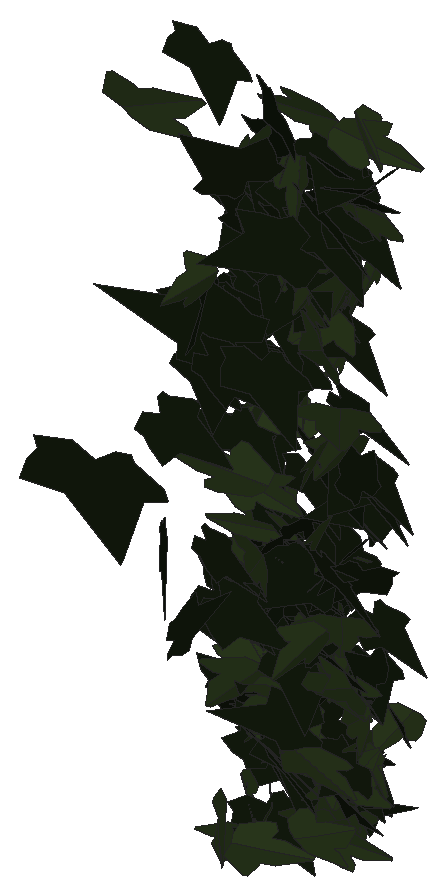
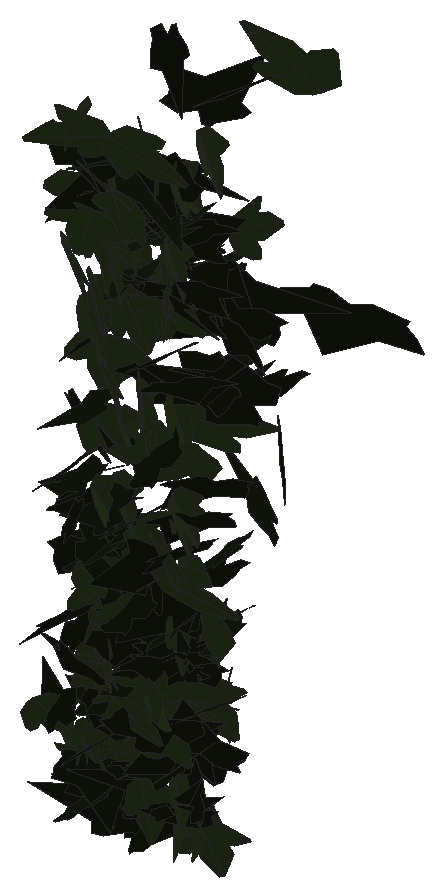
# SketchUp Ruby script. Lengths in millimetres.
U = 1.mm
M = Sketchup.active_model
def pt(a) = Geom::Point3d.new(a.map { |v| v * U })
def face(e, loops, mat)
  f = e.add_face(loops[0].map { |a| pt(a) })
  loops[1..].each { |l| e.add_face(l.map { |a| pt(a) }).erase! }
  f.material = f.back_material = mat if mat
  f
end
# faces: each face lists its corners as indices into pts; further lists are holes
def faces(e, pts, list, mat = nil) = list.each { |f| face(e, (f[0].is_a?(Array) ? f : [f]).map { |l| l.map { |i| pts[i] } }, mat) }
# xy, xz, yz: faces in a plane at the given z, y or x. An outline is a flat list of corners, or four numbers for a rectangle; further outlines are holes
def ring(l) = l.size == 4 ? [[l[0], l[1]], [l[2], l[1]], [l[2], l[3]], [l[0], l[3]]] : l.each_slice(2).to_a
def flat(e, list, mat, &to3) = list.each { |f| face(e, (f[0].is_a?(Array) ? f : [f]).map { |l| ring(l).map { |u, v| to3.(u, v) } }, mat) }
def xy(e, z, list, mat = nil) = flat(e, list, mat) { |x, y| [x, y, z] }
def xz(e, y, list, mat = nil) = flat(e, list, mat) { |x, z| [x, y, z] }
def yz(e, x, list, mat = nil) = flat(e, list, mat) { |y, z| [x, y, z] }
def lines(e, pts, list) = list.each { |a, b| e.add_line(pt(pts[a]), pt(pts[b])) }
# prism: a flat outline (further loops are holes) pulled along v
def prism(e, loops, v, mat = nil)
  f = face(e, loops, mat); d = Geom::Vector3d.new(v.map { |x| x * U })
  f.pushpull(f.normal.samedirection?(d) ? d.length : -d.length)
end
def box(e, o, s, mat = nil) = prism(e, [[o, [o[0] + s[0], o[1], o[2]], [o[0] + s[0], o[1] + s[1], o[2]], [o[0], o[1] + s[1], o[2]]]], [0, 0, s[2]], mat)
def at(x, y, z, deg = 0) = Geom::Transformation.translation(pt([x, y, z])) * Geom::Transformation.rotation(ORIGIN, Z_AXIS, deg.degrees)
def axes(o, x, y, z) = Geom::Transformation.new([*x, 0, *y, 0, *z, 0, *pt(o).to_a, 1])
def part(name) = M.definitions.add(name)
# library, detail: a bought-in or finely detailed component or shape, given as its bounding box
def library(name, o, s) = part(name).tap { |d| box(d.entities, o, s) }
def detail(e, o, s) = box(e.add_group.entities, o, s)
def put(e, d, t, mat = nil) = e.add_instance(d, t).tap { |i| i.material = mat if mat }
def group(e, t, mat = nil) = e.add_group.tap { |g| g.transformation = t; g.material = mat if mat }.entities
root = M.entities
M.materials.add("efeu1").color = [18, 25, 13]
M.materials.add("efeu2").color = [43, 57, 29]
c1 = part("ivyleaf_9")
p = [[39.1,54.8,31.7],[34.5,51.8,30.2],[-5.3,25.2,17.3],[-17.9,28.3,20.9],[-21.6,21.7,17],[-20.2,4.3,5.3],
  [-22.9,-0.3,2.5],[-17.1,-4,-0.6],[-2,-2.1,-1.2],[-0.7,-15.4,-10.1],[16.6,-22.3,-16.7],[21.1,-15.1,-12.5],
  [32.7,-10.7,-11],[46.1,-1.8,-6.6],[30.8,11.2,3.8]]
faces(c1.entities,p,[[0,1,2,3,4,5,6,7,8,9,10,11,12,13,14]],"efeu1")
c2 = part("ivyleaf_10")
p = [[0,12.8,-0.8],[-1.5,51.3,-10.9],[-4.9,51,-11.6],[-13.6,26.5,-7.3],[-13.2,15.9,-4.6],[-21.1,19.3,-7.2],
  [-29.5,16.3,-8.3],[-29.2,8.3,-6.2],[-19.7,-9.8,0.5],[-7.6,-13,4],[1,-12.2,5.8],[-0.4,51.1,-11.1],
  [-1.5,51.1,-10.9],[1,-12.4,5.9],[16.9,-12.4,3.5],[35.1,9.1,-5.1],[35,12.9,-6.1],[20.5,16.4,-4.9],
  [15.8,15,-3.8],[15.3,27.6,-7.1],[12.8,31.3,-7.8]]
faces(c2.entities,p,[[0,1,2,3,4,5,6,7,8,9,10],[11,12,0,13,14,15,16,17,18,19,20]],"efeu2")
put(root,c1,axes([2891.1,869.5,1834.3],[-0.39731,-0.86829,0.31305],[0.04934,-0.32634,-0.88788],[1.75596,-0.18729,0.09578]))
put(root,c1,axes([2913.8,889.4,2372.3],[-1.52857,-0.57999,0.09291],[-0.15236,-0.04783,-0.99065],[1.10747,-0.8071,-0.00805]))
put(root,c1,axes([2889.1,813.4,2596.7],[-0.24344,-1.08437,0.12243],[0.03551,-0.12542,-1.09139],[2.07658,-0.12498,0.03302]))
put(root,c1,axes([2894.1,816.4,2302],[-1.21063,0.10357,-0.85726],[1.61274,-0.12983,-0.64446],[-0.31595,-1.05956,-0.00482]))
put(root,c1,axes([2903.3,896.4,2257.5],[-0.95769,-0.82989,0.02779],[-0.00085,-0.03222,-0.97039],[1.58033,-0.50294,0.01632]))
put(root,c1,axes([2905.3,859.3,1887.5],[0.17862,0.16673,1.04725],[-0.99199,-0.90834,0.19133],[1.75762,-0.5296,0.00155]))
put(root,c1,axes([2892.5,885.9,2087.2],[-0.4143,-0.82836,-0.40314],[0.25079,0.38199,-0.85604],[1.73529,-0.25297,0.02747]))
put(root,c1,axes([2894.2,900.4,1922],[-0.27591,-0.949,0.24615],[0.02313,-0.25055,-0.95879],[1.86575,-0.13723,0.04829]))
put(root,c1,axes([2866.6,820.1,2211.3],[0.64718,0.02572,1.00838],[1.91908,-0.03717,-0.33909],[0.05141,1.06352,-0.03623]))
put(root,c1,axes([2882,887.7,1742.6],[0.27256,-0.23238,-0.90435],[1.61402,-0.35047,0.22435],[-0.7436,-0.84589,0.15549]))
put(root,c2,axes([2939.3,868.2,1982.5],[0.59483,0.01615,-0.956],[-1.78438,0.20243,-0.3031],[0.35688,0.98521,0.07795]))
put(root,c2,axes([2910.5,885.7,2095.9],[0.17575,-0.92048,0.18319],[0.01931,-0.18308,-0.92507],[1.78611,0.09255,-0.00802]))
put(root,c2,axes([2879.3,701.6,2567.1],[-1.49145,-0.22161,0.85578],[1.56205,0.24244,0.81436],[-0.625,1.13477,-0.00685]))
put(root,c1,axes([2906.2,856.6,1774.9],[-1.41852,0.16412,0.5402],[0.86669,-0.35408,0.73589],[0.63516,0.84969,0.20232]))
put(root,c1,axes([2885.8,791.7,2255.2],[1.01926,-0.9246,-0.15239],[-0.116,0.14079,-1.06836],[1.77966,0.53872,0.01765]))
put(root,c1,axes([2893.3,850.6,2114.9],[-0.09847,-0.77447,-0.6047],[0.38727,0.58397,-0.76533],[1.82952,-0.1653,0.12946]))
put(root,c2,axes([2916.8,880.2,1733.2],[-0.04261,-0.81588,-0.30481],[0.01402,0.30473,-0.81619],[1.65756,-0.02355,-0.00093]))
put(root,c2,axes([2886.3,860,1941.3],[-0.9887,0.16153,-0.83821],[1.37631,-0.43811,-0.53261],[-0.86327,-0.88348,0.11086]))
put(root,c2,axes([2918,879.8,1935.2],[-0.167,-0.87943,-0.25482],[-0.01447,0.25667,-0.88322],[1.74251,-0.08215,-0.03175]))
put(root,c1,axes([2890.3,843.1,1913.8],[0.41806,-0.90955,0.34178],[0.24813,-0.31964,-0.93444],[1.83252,0.25078,0.04856]))
put(root,c1,axes([2924,874.4,1697.5],[-1.00334,-0.63291,0.45548],[0.65619,0.30394,0.8214],[-1.33109,0.6269,0.0616]))
put(root,c2,axes([2922.3,873.5,2081.6],[-0.01062,-0.9292,-0.11369],[-0.05992,0.11381,-0.92867],[1.78063,-0.00171,-0.03193]))
put(root,c2,axes([2935.9,830.1,1821.4],[-0.92639,-0.77642,0.61795],[-0.53165,-0.55324,-0.91516],[1.8122,-0.55921,0.04741]))
put(root,c1,axes([2969.9,747,2288.3],[-0.92588,0.13082,1.16642],[-2.18444,0.21109,-0.50238],[-0.46726,-1.24605,0.03736]))
put(root,c1,axes([2907.2,789.2,2205],[-0.18215,-0.90601,0.46397],[0.04865,-0.46801,-0.90862],[1.93666,-0.07346,0.06647]))
put(root,c1,axes([2905.1,881.6,2041.2],[0.27827,-0.82186,-0.40667],[0.01821,0.41315,-0.83152],[1.74509,0.12674,0.07352]))
put(root,c2,axes([2928.1,845.2,1835.7],[0.54287,1.01027,0.21761],[-0.1101,-0.20978,1.04977],[1.96376,-0.29104,-0.0013]))
put(root,c2,axes([2927.4,877.9,2407.9],[0.25726,-0.99131,-0.1389],[-0.01361,0.1392,-1.00042],[1.90505,0.13486,0.01161]))
put(root,c1,axes([2905.4,713.9,2182.9],[0.74174,-0.54202,-0.89548],[-0.34457,0.90623,-0.62732],[1.96214,0.36404,0.22835]))
put(root,c1,axes([2906.2,803.3,1921],[0.72559,-0.682,-0.51529],[-0.14278,0.53534,-0.76406],[1.62054,0.35253,0.1634]))
put(root,c1,axes([2908,866.6,1769.9],[0.69712,-0.81594,-0.43061],[-0.25962,0.41031,-0.89352],[1.73658,0.38889,0.03928]))
put(root,c2,axes([2915.6,847.9,1664.7],[-0.3388,0.37149,-0.87717],[0.4574,-0.84597,-0.40705],[-1.75432,-0.29231,0.06327]))
put(root,c2,axes([2942.4,803.6,1634.4],[-1.06652,-0.65111,0.2249],[-0.28252,-0.16897,-0.85905],[1.28023,-0.57971,-0.00221]))
put(root,c1,axes([2923.4,901.3,1904],[-0.62312,-0.90946,-0.21573],[0.08326,0.21342,-0.96612],[1.77697,-0.32892,-0.03038]))
put(root,c1,axes([2926.4,778.9,2315],[-0.28877,0.10468,-1.0156],[1.20542,-0.79566,-0.17664],[-1.52405,-0.64915,0.05272]))
put(root,c1,axes([2914.5,781.9,1996.5],[0.99589,-0.6204,-0.48779],[-0.34731,0.4743,-0.79899],[1.4613,0.53554,0.14254]))
put(root,c1,axes([2907.2,819.7,2225.1],[1.71698,-0.32944,0.02387],[0.04164,-0.00967,-0.96042],[0.62726,0.90242,-0.00158]))
put(root,c2,axes([2933.5,857.3,2483.9],[0.35917,-0.88894,0.47616],[0.18964,-0.46562,-0.90875],[1.90986,0.21341,0.00069]))
put(root,c1,axes([2910.2,787.2,2300.9],[-0.51577,-0.50327,-0.93319],[0.98436,0.77806,-0.56981],[1.76148,-0.58216,0.04518]))
put(root,c1,axes([2953,850.8,1797.2],[0.55805,0.45519,-0.70167],[-0.94938,-0.50164,-0.53389],[-1.2777,0.57155,0.09024]))
put(root,c1,axes([2944.4,894.2,1704.1],[-1.22441,-0.61132,0.22429],[-0.2908,-0.16477,-0.88736],[1.2047,-0.6611,0.01376]))
put(root,c1,axes([2912.3,841.7,1772.4],[1.58911,0.39922,0.37226],[0.62163,0.17967,-0.92529],[-0.83236,0.89637,0.01967]))
put(root,c1,axes([2915.9,886.4,1938.8],[0.63248,-0.87598,-0.00707],[-0.00131,0.0073,-0.9369],[1.66722,0.33232,0.00195]))
put(root,c2,axes([2937.9,884.2,2028.1],[1.1876,-0.68664,0.00438],[-0.01376,-0.01249,-0.92772],[1.30676,0.62389,-0.01375]))
put(root,c2,axes([2940.7,875.9,2380.1],[0.66023,-0.84828,-0.3577],[0.04379,0.39012,-0.90286],[1.75156,0.31,0.1574]))
put(root,c1,axes([2923.2,886.8,2008.7],[0.32724,-0.89909,-0.13673],[-0.09238,0.12988,-0.91509],[1.72836,0.17717,-0.02302]))
put(root,c1,axes([2938.6,854.2,2425.1],[-1.08727,-0.85782,-0.06748],[0.06601,0.05797,-1.03064],[1.63631,-0.57233,-0.00326]))
put(root,c1,axes([2969,884.4,1782.9],[0.03609,0.05867,0.96721],[-1.84418,0.00306,0.01881],[-0.00365,-0.96739,0.05871]))
put(root,c2,axes([2940.3,872.7,2327.7],[-0.74477,0.84013,-0.29287],[-0.15829,-0.35309,-0.90174],[-1.68589,-0.33799,0.21405]))
put(root,c1,axes([2918.7,866,1891.3],[-0.29974,-0.47439,-0.79773],[0.88279,0.66062,-0.48443],[1.53001,-0.4741,0.12322]))
put(root,c1,axes([2970.1,817.7,2390],[0.43909,-0.18701,0.99494],[-1.43483,0.64931,0.29686],[-1.28591,-0.78837,0.00849]))
put(root,c2,axes([2945.1,732.1,2363.5],[0.01931,-0.17762,1.12447],[0.26196,-1.11607,-0.17754],[2.15073,0.13753,0.01153]))
put(root,c1,axes([2929.9,563,2198.1],[-1.61713,-0.61122,-0.89076],[1.32358,0.55774,-1.04609],[1.57333,-1.09743,-0.03553]))
put(root,c2,axes([2950,790.8,2495.5],[0.28401,-1.08152,-0.05502],[-0.01306,0.05459,-1.09177],[2.06098,0.14939,0.00066]))
put(root,c1,axes([2938.3,861.6,2426.8],[-0.48157,-0.72232,0.64363],[-0.04634,-0.66031,-0.75062],[1.84071,-0.2056,0.14949]))
put(root,c2,axes([2952.5,816.4,1975.6],[1.12327,-0.60662,-0.52893],[-0.24574,0.57604,-0.80473],[1.51191,0.54431,0.26217]))
put(root,c1,axes([2932.6,870.9,1961.6],[1.60439,0.42216,0.07732],[0.13015,0.03613,-0.9428],[-0.80639,0.84577,0.00168]))
put(root,c1,axes([2964.1,847.7,2316.6],[-1.66101,-0.40517,0.12381],[-0.20649,-0.06032,-0.96217],[0.77944,-0.87942,0.00895]))
put(root,c1,axes([2936.5,901.3,1767.2],[-0.12874,-0.88522,0.12997],[0.02897,-0.13146,-0.88745],[1.70256,-0.0647,0.02493]))
put(root,c1,axes([2958.7,837.1,1895.6],[0.15748,0.21127,0.97971],[0.15262,0.97849,-0.21778],[-1.90133,0.09604,0.06366]))
put(root,c1,axes([2975.4,870.9,2345.9],[-1.82963,0.16596,0.05366],[-0.11269,-0.0278,-0.97484],[-0.31223,-0.96244,0.03741]))
put(root,c1,axes([2941.6,880.2,1873.7],[-0.75603,-0.84554,-0.33297],[0.31293,0.29052,-0.9339],[1.70097,-0.42927,0.02382]))
put(root,c2,axes([2956.6,835,2182],[-0.01482,-0.95669,-0.01264],[0.00028,0.01263,-0.95672],[1.82093,-0.00779,0.00004]))
put(root,c1,axes([2915.9,882.2,1931.9],[1.19246,-0.57058,0.56143],[0.84071,-0.34812,-0.84677],[1.27049,0.76589,0.03338]))
put(root,c2,axes([2968.6,839.7,1796.5],[-1.38421,-0.43098,0.27772],[-0.48297,-0.11622,-0.84495],[0.84788,-0.7698,-0.02792]))
put(root,c1,axes([2975.7,859.5,2464.9],[-0.04149,0.95328,0.2503],[-0.47778,0.23673,-0.92348],[-1.81392,-0.08416,0.23751]))
put(root,c1,axes([2936.2,674.5,2061.2],[-0.42606,0.10081,-1.19076],[1.94447,-0.61225,-0.24391],[-1.17971,-1.04555,0.02801]))
put(root,c2,axes([2960.8,884.1,1714.8],[-0.48863,-1.00139,-0.13294],[0.02559,0.13376,-1.03358],[1.92239,-0.25631,-0.02003]))
put(root,c2,axes([2960.6,827.3,1662.8],[0.2008,-0.67668,-0.72818],[-0.06892,0.72917,-0.68284],[1.89063,0.09845,0.05245]))
put(root,c2,axes([2988,756.1,2116.8],[0.5094,0.20594,1.03616],[-1.52872,-0.65461,0.33759],[1.30594,-0.84661,-0.00898]))
put(root,c2,axes([2942,878.5,1815.1],[0.50922,-0.89635,-0.51151],[0.39961,-0.47009,0.9336],[-1.92308,-0.33503,0.05856]))
put(root,c2,axes([2939.7,840.2,2334.2],[1.25596,-0.82122,-0.43743],[0.49461,-0.35225,1.05338],[-1.70035,-0.70905,-0.01669]))
put(root,c2,axes([2943.9,875.8,1785.5],[-1.32639,-0.21557,-0.487],[1.00377,-0.16798,-0.68041],[0.14075,-0.83346,0.26309]))
put(root,c1,axes([2946.4,870.1,2265],[-0.03782,-0.96097,0.02757],[0.00901,-0.02767,-0.96116],[1.82964,-0.01973,0.0053]))
put(root,c2,axes([2954.6,856.7,2314.9],[-1.25085,-0.58846,-0.40322],[0.66444,0.21278,-0.87959],[1.18396,-0.74112,0.06763]))
put(root,c2,axes([2992.6,877.9,2517.9],[0.6275,0.14151,-0.93722],[-1.65586,0.4389,-0.23981],[0.71575,0.89132,0.26688]))
put(root,c1,axes([2958.3,873.9,2405.7],[-0.84119,-0.66489,0.62532],[-0.02533,-0.69,-0.74308],[1.73695,-0.33206,0.292]))
put(root,c2,axes([2945.8,880,1869.9],[-0.51172,0.2972,-0.79231],[0.70467,-0.70623,-0.39056],[-1.44818,-0.44866,0.08993]))
put(root,c2,axes([2984.3,866.4,1755.7],[1.20829,0.02719,-0.70769],[-1.34303,-0.05628,-0.63522],[-0.11425,0.94907,-0.01739]))
put(root,c1,axes([2938.5,887.5,2135.3],[0.45383,-0.82155,0.67292],[0.27367,-0.65834,-0.85471],[2.00251,0.27616,-0.0357]))
put(root,c2,axes([2986.6,896.6,1819.3],[-1.39375,0.16904,0.49146],[-0.96731,-0.41029,-0.61623],[0.20659,-0.7807,0.43027]))
put(root,c1,axes([2958.4,860.8,1988],[-0.13058,0.61433,-0.87602],[-0.38116,0.85494,0.61523],[2.00036,0.20301,0.06004]))
put(root,c2,axes([2961.8,859.7,2130.9],[1.24869,0.74984,-0.18852],[0.23478,0.14256,0.99636],[1.45266,-0.6676,0.00102]))
put(root,c1,axes([2944.6,824.1,1745.7],[1.47133,-0.4333,-0.04863],[-0.06568,0.03787,-0.88608],[0.82723,0.77368,0.01614]))
put(root,c2,axes([2958.2,889.1,1848.4],[-1.36965,0.53653,-0.33194],[0.49506,-0.20642,-0.89759],[-1.09393,-0.76517,0.00939]))
put(root,c2,axes([2987.2,838.3,1801.9],[1.46618,-0.01339,-0.6543],[-1.24384,0.03664,-0.77025],[0.06456,1.01007,0.01927]))
put(root,c2,axes([2971.1,851,2478.1],[0.46098,-0.85358,-0.45244],[0.14235,0.48161,-0.86857],[1.83311,0.17725,0.18123]))
put(root,c1,axes([2953.6,759.5,1947.3],[0.69026,-0.51266,-0.89681],[-0.35399,0.90254,-0.59115],[1.93387,0.34819,0.21189]))
put(root,c2,axes([2988.7,839.8,1825.9],[1.07037,-0.15638,-0.72137],[-0.85781,0.64544,-0.49131],[1.11249,0.64814,0.31522]))
put(root,c2,axes([2979.3,882.9,2316.3],[-0.65187,-0.89122,0.22495],[-0.00912,-0.23832,-0.95151],[1.74935,-0.33334,0.07886]))
put(root,c1,axes([2946.1,858.3,1754.3],[1.5578,-0.6342,0.03381],[0.05705,-0.01651,-1.03545],[1.20737,0.81905,0.0053]))
put(root,c1,axes([2938.2,866.7,2468.1],[0.48145,-0.35278,0.9231],[1.26669,-0.64352,-0.42833],[1.39023,0.70851,0.07058]))
put(root,c1,axes([2960.7,827.3,1662],[-0.12138,-0.73332,-0.67601],[0.10284,0.67386,-0.73608],[1.89541,-0.08352,-0.00335]))
put(root,c1,axes([2971.3,840,2223.1],[-1.17309,-0.68009,-0.36267],[0.46785,0.26666,-0.91784],[1.39027,-0.66358,0.00286]))
put(root,c1,axes([2965,835,2410.2],[-0.16036,-0.99949,0.10595],[-0.01359,-0.10573,-1.00304],[1.91285,-0.08454,0.00175]))
put(root,c2,axes([2974.5,843.1,2333.9],[0.87307,-0.91889,0.39791],[0.31134,-0.36302,-1.02693],[1.88015,0.48681,-0.01472]))
put(root,c2,axes([2954.6,839.1,1782.1],[-0.91262,-0.19549,-0.72079],[1.41897,-0.07556,-0.47551],[0.08255,-0.86242,0.20505]))
put(root,c2,axes([2988,845.2,2326.9],[1.15911,-0.59378,-0.46952],[-0.37419,0.45785,-0.83406],[1.39125,0.61785,0.16685]))
put(root,c2,axes([2986.6,893.7,1947],[0.65448,0.66767,-0.50509],[-0.62322,-0.39526,-0.74545],[-1.46642,0.46598,0.09139]))
put(root,c1,axes([2994.8,859.2,1638.5],[0.10725,-0.81228,0.5586],[-0.05895,0.55778,0.8142],[-1.87528,-0.06399,0.00635]))
put(root,c1,axes([2997.9,894.6,1911.9],[-0.37518,0.05449,-0.90117],[0.03415,-0.92199,-0.05968],[-1.71791,-0.03023,0.19562]))
put(root,c1,axes([2998.8,738.4,2503.6],[0.48419,0.1856,1.10471],[-1.86271,-0.51423,0.31179],[1.03707,-1.01028,0.04424]))
put(root,c2,axes([2987.5,852,2181],[0.85105,-0.71012,-0.55555],[-0.12,0.59398,-0.80999],[1.71176,0.3947,0.21943]))
put(root,c1,axes([3003.3,848.2,1961.5],[-1.93823,0.03309,-0.08224],[0.15628,-0.00522,-1.01894],[-0.06357,-1.02171,0.00254]))
put(root,c1,axes([2968.7,892.8,2060.2],[0.21642,-0.91598,-0.09853],[-0.04359,0.09643,-0.92295],[1.75281,0.1155,-0.01079]))
put(root,c1,axes([3023.1,863.3,1778.7],[-0.50658,-0.26153,-0.9192],[-1.29413,-0.61865,0.37292],[-1.27806,0.73009,-0.01327]))
put(root,c1,axes([2963.4,904.9,1946.8],[0.35783,-0.66422,0.67362],[0.4867,-0.62555,-0.68819],[1.73344,0.31275,0.05417]))
put(root,c2,axes([2986.2,886.9,2442.4],[-1.5054,0.56761,-0.16698],[0.21031,-0.13215,-0.97265],[-1.10623,-0.79754,0.04232]))
put(root,c2,axes([2968.9,784.2,2088.8],[0.89953,0.38009,0.74129],[0.74883,0.64938,-0.58383],[-1.39748,0.59262,0.16431]))
put(root,c1,axes([3022.4,812.7,1790.4],[-1.13107,0.04,0.67268],[-1.26972,-0.1613,-0.57982],[0.18071,-0.88299,0.13639]))
put(root,c1,axes([2969.3,845.6,1710.4],[0.33191,-0.68198,0.53825],[0.33984,-0.50913,-0.70294],[1.6182,0.24681,0.03722]))
put(root,c1,axes([2987.1,831.1,2334.1],[-0.74758,-0.89701,0.42334],[-0.08315,-0.43924,-0.97124],[1.88594,-0.37494,0.12499]))
put(root,c2,axes([2997.7,842,2201.6],[0.07837,-0.79093,-0.60404],[-0.04702,0.60356,-0.79199],[1.89349,0.04773,0.00533]))
put(root,c1,axes([2974.8,651.1,1957.8],[0.0533,1.00742,0.6907],[-0.03764,-0.69042,1.00781],[2.32438,-0.03428,0.00048]))
put(root,c2,axes([2969.8,777.9,1640],[-0.27252,-0.3257,-1.00644],[1.46045,0.66708,-0.32506],[1.38575,-0.76709,0.14465]))
put(root,c1,axes([2971.6,852,2324.6],[0.89821,-0.77385,-0.56417],[-0.13611,0.59872,-0.88107],[1.81755,0.42726,0.21283]))
put(root,c1,axes([2986.1,895.9,2313.5],[-0.54129,-0.89267,0.27207],[0.12185,-0.30242,-0.92532],[1.7719,-0.2519,0.14674]))
put(root,c1,axes([2991.9,856,1730.1],[-0.77135,-0.94033,-0.05742],[0.06259,0.04835,-1.0239],[1.79188,-0.40647,0.01105]))
put(root,c2,axes([2986.7,855.7,1735.5],[-0.72638,0.43036,-0.66955],[0.54812,-0.61757,-0.56112],[-1.41218,-0.46107,0.12661]))
put(root,c2,axes([3000.8,888.8,2367.3],[0.54894,-0.94608,-0.0449],[0.1382,0.06889,-0.98502],[1.79731,0.28366,0.08946]))
put(root,c1,axes([2988,878.2,2343.8],[-0.00803,-0.88668,0.46932],[0.10194,-0.46885,-0.88532],[1.90662,0.02133,0.04931]))
put(root,c1,axes([3029.7,886.1,2468.5],[-1.6619,0.46178,-0.11175],[0.1337,-0.10576,-0.98596],[-0.8943,-0.87396,0.06026]))
put(root,c1,axes([3002.9,842.4,1861.1],[-0.76699,0.9419,-0.05473],[-0.0414,0.05022,1.02449],[1.79517,0.40359,0.00025]))
put(root,c1,axes([3027.7,760.1,2588.4],[0.65597,0.02289,-1.06433],[-1.93656,0.33599,-0.32228],[0.59568,1.0671,0.12431]))
put(root,c1,axes([2997.6,833.3,1848.3],[-0.20396,-0.96755,0.14437],[-0.03005,-0.1435,-0.97346],[1.86158,-0.10832,0.0001]))
put(root,c1,axes([3002.4,841.5,2428.2],[-0.55554,-0.91853,0.38644],[-0.04983,-0.39547,-0.95977],[1.8959,-0.27954,0.08801]))
put(root,c1,axes([2989.9,691.8,2295.2],[1.25456,-0.61663,-0.69147],[-0.45169,0.70792,-0.85755],[1.70443,0.64148,0.2817]))
put(root,c2,axes([3012.9,889.5,2234.1],[0.95369,-0.81653,-0.07831],[-0.03916,0.07922,-0.95773],[1.56066,0.50095,0.02382]))
put(root,c2,axes([3015.1,831.1,1773.9],[-0.92127,0.85664,0.25934],[-0.27186,0.21712,-0.9838],[-1.6816,-0.50442,0.01697]))
put(root,c2,axes([3018.8,864,2442.7],[0.45273,-0.94099,-0.26327],[-0.07909,0.26097,-0.97033],[1.85799,0.2404,0.02284]))
put(root,c2,axes([3020.1,879.6,1887.1],[0.54692,-0.83674,-0.59524],[-0.13772,0.60007,-0.87846],[1.94945,0.27714,0.10493]))
put(root,c1,axes([3012.2,863.1,2306.1],[-0.89642,-0.65424,0.61164],[-0.05632,-0.67932,-0.74943],[1.70362,-0.36672,0.29706]))
put(root,c1,axes([3028.9,808.4,2407],[-0.94139,0.78891,-0.58113],[0.5717,-0.49754,-0.93112],[-1.77504,-0.57864,0.00831]))
put(root,c1,axes([3023.9,878.3,1817.9],[-0.35724,0.45805,-0.73656],[0.42574,-0.70256,-0.49391],[-1.59494,-0.29013,0.03314]))
put(root,c2,axes([3012.3,822.1,2321.5],[-1.18709,0.74173,-0.10148],[0.11085,-0.08361,-0.96908],[-1.42049,-0.62638,0.00918]))
put(root,c2,axes([3000.6,848.2,2358.7],[0.17859,-0.52453,0.8809],[1.02984,-0.726,-0.48994],[1.65733,0.50765,0.20952]))
put(root,c2,axes([3015.8,896.4,2077.9],[0.40621,-0.82322,0.38631],[0.21075,-0.37033,-0.85034],[1.71781,0.2401,0.01297]))
put(root,c2,axes([3035.4,861.4,1665],[-0.43285,0.00124,-0.85488],[-1.09814,-0.65295,0.15256],[-1.20052,0.59682,0.16868]))
put(root,c2,axes([2998.4,697.5,1725.2],[0.27551,-0.45523,1.14308],[1.32372,-0.91915,-0.45413],[1.93164,0.69481,0.14817]))
put(root,c2,axes([3021.2,840,1667.8],[-1.08608,-0.66814,-0.14881],[-0.1492,-0.12867,0.87835],[-1.29418,0.57553,0.02362]))
put(root,c2,axes([3004.6,820,2481.3],[1.25528,-0.7004,0.64569],[0.85062,-0.46603,-0.96206],[1.60109,0.79672,0.00489]))
put(root,c1,axes([3052.8,760.6,2423.8],[-1.75996,-0.2032,0.46252],[-0.85071,-0.12042,-0.9466],[0.448,-1.02692,0.01949]))
put(root,c1,axes([3010.3,892.6,1980],[-0.069,-0.92196,0.14939],[-0.03228,-0.14883,-0.92261],[1.77727,-0.0385,-0.01096]))
put(root,c1,axes([3032.4,880.7,1721.8],[0.48025,0.8284,-0.24232],[-0.17911,-0.22455,-0.86566],[-1.63289,0.26828,0.02368]))
put(root,c1,axes([2998.4,886.8,2060.2],[1.05607,-0.74253,0.11901],[0.13915,-0.09393,-0.92696],[1.42444,0.55968,0.00232]))
put(root,c2,axes([3026.9,834.5,2132.8],[0.50886,-1.04337,0.12862],[0.06514,-0.124,-1.07708],[1.99972,0.26954,0.00236]))
put(root,c1,axes([3003.5,885.6,1716.9],[-0.32939,-0.60211,-0.67608],[0.80264,0.55545,-0.60265],[1.52465,-0.4225,0.1712]))
put(root,c2,axes([3038.3,834.1,2300.8],[1.69906,-0.27797,-0.42476],[-0.75567,0.15304,-0.93466],[0.60194,0.97672,0.02557]))
put(root,c2,axes([3033.8,883.8,2332.6],[0.73948,-0.84191,-0.32221],[-0.10917,0.32706,-0.92377],[1.71219,0.38447,0.08026]))
put(root,c1,axes([3004.8,895.4,1821.5],[0.37141,-0.73959,0.47212],[0.49883,-0.41244,-0.75444],[1.59369,0.30146,0.12611]))
put(root,c2,axes([3032.8,895.4,2306.8],[0.01855,-0.96424,0.1374],[0.10184,-0.13667,-0.96291],[1.85088,0.01719,0.0516]))
put(root,c2,axes([3033.9,873.4,2377.1],[0.96631,-0.79118,-0.36436],[-0.08472,0.39762,-0.92544],[1.65562,0.48212,0.16531]))
put(root,c1,axes([3016.5,822.7,2390.3],[0.01012,-1.01861,-0.0839],[0.01215,0.08393,-1.0186],[1.94514,0.00477,0.0068]))
put(root,c1,axes([3000.8,853.3,1863.2],[0.39883,-0.48225,0.93208],[0.79863,-0.83269,-0.52517],[1.83069,0.46832,0.02604]))
put(root,c2,axes([3044.3,872.1,1831.2],[-1.12419,0.49166,0.45198],[-0.63112,0.30784,-0.76824],[-1.10328,-0.67707,-0.02108]))
put(root,c2,axes([3040.9,885.2,1966],[-0.20954,-0.73271,0.51048],[-0.17092,-0.50265,-0.74084],[1.69094,-0.1416,-0.01163]))
put(root,c2,axes([3037.5,867.2,2317.6],[-0.15472,-0.95089,-0.21279],[0.0719,0.21029,-0.95417],[1.8531,-0.08755,0.01926]))
put(root,c2,axes([3040.1,822.1,2360.2],[-0.19077,-0.90204,0.4628],[-0.0159,-0.4643,-0.90678],[1.92946,-0.09301,0.03829]))
put(root,c2,axes([3041,826,2048.2],[0.20118,-0.97124,-0.12365],[-0.01706,0.1234,-0.97696],[1.8633,0.106,0.00441]))
put(root,c2,axes([3034.9,869.1,1853.1],[0.96021,-0.84163,0.19293],[0.17325,-0.17036,-0.98122],[1.63417,0.51258,-0.00934]))
put(root,c1,axes([3034.2,868.7,2476.7],[-0.92773,-0.78571,0.4364],[0.06144,-0.51144,-0.88475],[1.70942,-0.40803,0.26864]))
put(root,c1,axes([3006.4,856.9,1661.8],[0.58429,0.04655,0.93936],[1.74684,0.20083,-0.30992],[-0.39066,0.96764,0.01914]))
put(root,c2,axes([3050.2,854.2,2139.3],[-0.50066,-0.90601,0.45963],[-0.20979,-0.44653,-0.94328],[1.9221,-0.28473,0.01677]))
put(root,c1,axes([3047.9,876.6,1997.3],[-0.84798,0.32587,-0.73762],[0.70559,-0.6656,-0.51799],[-1.36292,-0.54733,0.19076]))
put(root,c2,axes([3042.4,884.3,2411.9],[-1.86099,0.10966,-0.10936],[0.15219,-0.24119,-0.95685],[-0.25243,-0.9539,0.22936]))
put(root,c1,axes([3006.5,855.2,1693.4],[0.61739,-0.51928,0.8931],[0.8907,-0.76067,-0.61227],[1.75287,0.56943,-0.00345]))
put(root,c1,axes([3020.5,838.3,2442.7],[1.35304,0.48786,0.56603],[0.85914,0.34221,-0.86193],[-1.13335,0.84184,0.02236]))
put(root,c1,axes([3039.5,892,1982.3],[-0.59361,-0.57141,0.66335],[-0.19134,-0.67615,-0.62971],[1.65527,-0.28308,0.1651]))
put(root,c2,axes([3048.5,845.7,1914.7],[-1.38094,-0.62656,-0.03145],[0.04415,0.02126,-0.95867],[1.19316,-0.72596,-0.00093]))
put(root,c1,axes([3028.9,908,1683],[-0.08183,-0.80942,0.46465],[0.06545,-0.4662,-0.80894],[1.77507,-0.02012,0.05125]))
put(root,c2,axes([3070.5,782.9,2292.3],[-1.02373,0.34428,0.90384],[-1.42866,0.50355,-0.63855],[-1.16074,-0.92342,-0.01122]))
put(root,c1,axes([3027.8,870.3,2269.8],[0.5221,-0.83287,-0.40037],[-0.17327,0.39125,-0.87628],[1.7502,0.28719,0.03268]))
put(root,c2,axes([3021.4,874.1,1669.8],[-0.01853,0.04122,0.89847],[1.37627,-0.53392,0.03233],[1.01785,0.72268,-0.02736]))
put(root,c1,axes([3046.7,885.2,2086.4],[-0.91102,-0.70634,0.46293],[-0.14605,-0.49354,-0.8324],[1.60066,-0.44705,0.18753]))
put(root,c2,axes([3052.2,848,1728.7],[-0.97942,-0.71785,0.2082],[0.08097,-0.28049,-0.86198],[1.42021,-0.47906,0.19272]))
put(root,c1,axes([3065.5,889.1,2047.8],[-0.93869,-0.36938,0.71696],[-1.00387,-0.48802,-0.61429],[1.1612,-0.7205,0.04852]))
put(root,c1,axes([3053.1,904,2025.5],[-0.07977,-0.03531,0.93001],[-0.73715,-0.84584,-0.04957],[1.61059,-0.38888,0.02337]))
put(root,c2,axes([3053.7,868.1,1753.4],[-0.35074,-0.84828,-0.40002],[0.24133,0.38139,-0.86719],[1.76857,-0.22027,0.039]))
put(root,c1,axes([3037.8,881.7,1745.4],[0.49551,-0.7735,-0.32739],[-0.18674,0.3124,-0.81612],[1.58762,0.27816,0.00618]))
put(root,c1,axes([3031.6,873.3,2176.1],[1.11692,-0.6803,-0.30129],[-0.12079,0.33656,-0.88357],[1.41088,0.56737,0.16287]))
put(root,c1,axes([3067.7,856.3,1981.6],[0.0925,0.54046,-0.76429],[-0.05811,-0.764,-0.54219],[-1.78059,0.05301,-0.02201]))
put(root,c1,axes([3038.6,720,2292],[-0.07239,-1.10121,-0.27767],[0.09081,0.27604,-1.10124],[2.15951,-0.04852,0.037]))
put(root,c1,axes([3040.9,826.5,2425.5],[-0.03487,-1.00316,-0.469],[-0.02018,0.4692,-1.00318],[2.10747,-0.0121,-0.01736]))
put(root,c2,axes([3082.4,813,1859.9],[-1.04619,0.19791,0.69322],[-1.29092,0.15335,-0.58164],[-0.46482,-0.87133,0.0551]))
put(root,c2,axes([3065.5,857.2,2430],[-1.8772,0.09088,0.02629],[-0.05338,-0.01793,-0.99031],[-0.17195,-0.98653,0.02042]))
put(root,c2,axes([3043.2,793.9,1766.6],[-1.32702,-0.07575,-0.56826],[1.08853,-0.03088,-0.69767],[0.07442,-0.89896,0.07185]))
put(root,c1,axes([3062.6,851.3,1741.4],[-0.55053,-0.58968,0.59581],[-0.44611,-0.54825,-0.65641],[1.53178,-0.3716,0.02297]))
put(root,c1,axes([3033.6,820.4,2445.2],[0.8992,-0.85734,0.3624],[0.27641,-0.33353,-0.9784],[1.74978,0.49327,-0.03168]))
put(root,c2,axes([3062.7,835.6,2357.7],[0.76201,-0.85297,-0.25877],[0.09096,0.30381,-0.92749],[1.69399,0.36738,0.1662]))
put(root,c1,axes([3036.8,832.1,1994.6],[0.98231,-0.85421,0.16966],[0.12608,-0.15814,-0.99773],[1.65269,0.51978,-0.02473]))
put(root,c2,axes([3059.7,871.7,2533.8],[-0.45304,0.98869,0.08205],[-0.03238,0.0803,-1.01694],[-1.88786,-0.23864,-0.00225]))
put(root,c2,axes([3063.1,888.8,2363.1],[1.03006,-0.82841,0.07096],[0.10313,-0.04934,-0.98937],[1.57903,0.54362,0.01833]))
put(root,c2,axes([3071.9,828,2362.5],[-0.35556,-1.01144,0.11178],[-0.00785,-0.1129,-1.02842],[1.93668,-0.18615,0.01635]))
put(root,c2,axes([3047.1,865.9,1706.7],[1.59604,-0.57924,-0.33432],[0.54013,-0.17731,1.0191],[-1.15257,-0.88521,0.01463]))
put(root,c2,axes([3077.4,841.1,1812],[0.926,-0.71146,-0.68703],[-0.47054,0.65386,-0.85221],[1.82257,0.53028,0.12904]))
put(root,c2,axes([3058.4,824.8,1853.8],[-1.53586,-0.17302,-0.36482],[0.69937,0.02312,-0.82382],[0.31842,-0.88532,0.04978]))
put(root,c1,axes([3043.8,888,2079],[0.69201,-0.84522,0.18301],[0.17058,-0.16063,-0.91993],[1.63704,0.37403,0.01849]))
put(root,c1,axes([3053.9,888.4,1852.9],[-0.88945,-0.24401,-0.71496],[1.42522,-0.03877,-0.47627],[0.18961,-0.85327,0.2261]))
put(root,c1,axes([3090.3,827.5,2109.5],[-0.03747,0.20976,0.97191],[-0.44024,0.94446,-0.20852],[-1.8404,-0.2302,0.03009]))
put(root,c2,axes([3077.3,807.1,2204],[-1.63353,-0.51145,-0.00686],[0.0119,0.00291,-0.99914],[0.97341,-0.85833,0.0007]))
put(root,c2,axes([3071.3,830.1,1679.7],[-0.83232,-0.78,-0.32184],[0.30305,0.27969,-0.89423],[1.57704,-0.46541,0.00198]))
put(root,c2,axes([3076.9,759.6,1944.1],[-0.22589,-0.72826,0.86435],[0.03837,-0.87033,-0.73053],[2.15075,-0.06096,0.10381]))
put(root,c2,axes([3037.1,831.3,1650.3],[-0.44961,0.00028,0.98914],[1.87413,0.09606,0.23516],[-0.17769,1.01242,-0.02259]))
put(root,c2,axes([3042.6,872.3,2512],[0.60041,0.25093,0.93435],[1.32012,0.62644,-0.40243],[-1.28357,0.76165,0.02317]))
put(root,c1,axes([3057.4,884.1,2098.2],[0.65474,-0.81704,-0.3168],[-0.23981,0.29068,-0.88651],[1.65046,0.36636,-0.00313]))
put(root,c1,axes([3055.3,853.3,2425.5],[0.30372,-0.87496,-0.4627],[0.0461,0.47199,-0.88417],[1.88318,0.12956,0.09627]))
put(root,c2,axes([3049.5,787.4,1673.9],[1.09547,-0.17565,-0.67433],[1.21874,-0.21157,0.60171],[-0.52297,-0.86097,-0.01029]))
put(root,c1,axes([3062,889.3,1909],[0.50005,-0.70515,-0.50734],[-0.14014,0.51005,-0.74705],[1.64735,0.25744,0.09045]))
put(root,c2,axes([3061.6,875.4,1735.8],[-0.38744,0.20119,-0.88456],[0.73478,-0.80114,-0.27107],[-1.56232,-0.42668,0.09188]))
put(root,c1,axes([3086.9,856.9,1849.6],[-0.02002,0.32907,0.84182],[-1.00833,-0.68432,0.26089],[1.39369,-0.49038,0.20084]))
put(root,c1,axes([3097.8,849.7,2484.9],[-0.64172,0.88364,-0.32096],[0.22808,-0.29779,-0.94577],[-1.77464,-0.3578,-0.00549]))
put(root,c1,axes([3066.5,906.6,1783.3],[-0.17033,-0.19387,0.91513],[0.25831,-0.91228,-0.17999],[1.7615,0.11503,0.11488]))
put(root,c2,axes([3091.2,902.8,1786.2],[-0.76728,-0.58171,0.56523],[-0.07813,-0.61576,-0.663],[1.5417,-0.32072,0.24771]))
